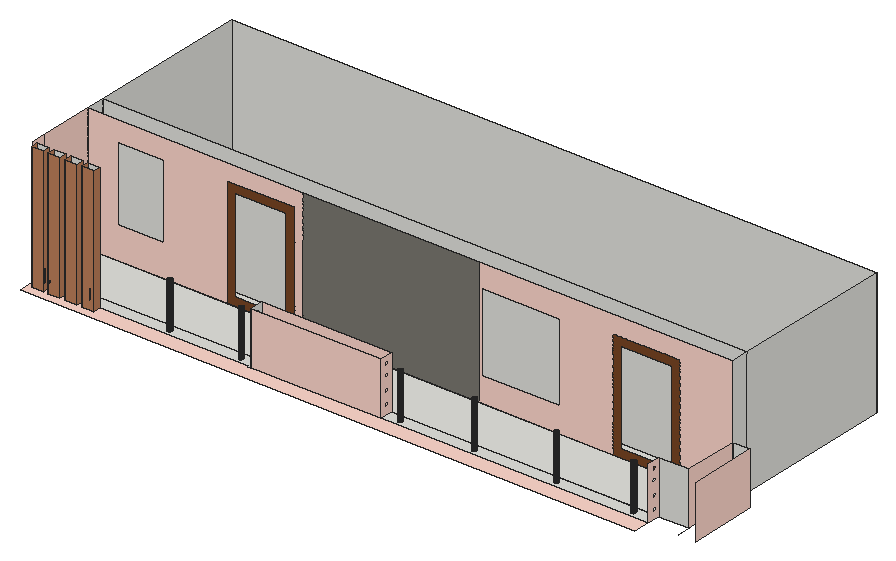
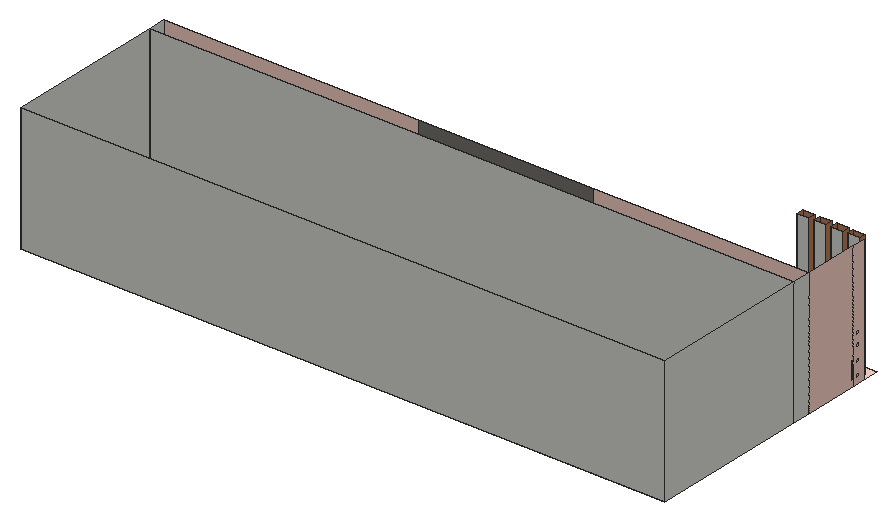
# SketchUp Ruby script. Lengths in inches.
U = 1.inch
M = Sketchup.active_model
def pt(a) = Geom::Point3d.new(a.map { |v| v * U })
def face(e, loops, mat)
  f = e.add_face(loops[0].map { |a| pt(a) })
  loops[1..].each { |l| e.add_face(l.map { |a| pt(a) }).erase! }
  f.material = f.back_material = mat if mat
  f
end
# faces: each face lists its corners as indices into pts; further lists are holes
def faces(e, pts, list, mat = nil) = list.each { |f| face(e, (f[0].is_a?(Array) ? f : [f]).map { |l| l.map { |i| pts[i] } }, mat) }
# xy, xz, yz: faces in a plane at the given z, y or x. An outline is a flat list of corners, or four numbers for a rectangle; further outlines are holes
def ring(l) = l.size == 4 ? [[l[0], l[1]], [l[2], l[1]], [l[2], l[3]], [l[0], l[3]]] : l.each_slice(2).to_a
def flat(e, list, mat, &to3) = list.each { |f| face(e, (f[0].is_a?(Array) ? f : [f]).map { |l| ring(l).map { |u, v| to3.(u, v) } }, mat) }
def xy(e, z, list, mat = nil) = flat(e, list, mat) { |x, y| [x, y, z] }
def xz(e, y, list, mat = nil) = flat(e, list, mat) { |x, z| [x, y, z] }
def yz(e, x, list, mat = nil) = flat(e, list, mat) { |y, z| [x, y, z] }
def lines(e, pts, list) = list.each { |a, b| e.add_line(pt(pts[a]), pt(pts[b])) }
# prism: a flat outline (further loops are holes) pulled along v
def prism(e, loops, v, mat = nil)
  f = face(e, loops, mat); d = Geom::Vector3d.new(v.map { |x| x * U })
  f.pushpull(f.normal.samedirection?(d) ? d.length : -d.length)
end
def box(e, o, s, mat = nil) = prism(e, [[o, [o[0] + s[0], o[1], o[2]], [o[0] + s[0], o[1] + s[1], o[2]], [o[0], o[1] + s[1], o[2]]]], [0, 0, s[2]], mat)
def at(x, y, z, deg = 0) = Geom::Transformation.translation(pt([x, y, z])) * Geom::Transformation.rotation(ORIGIN, Z_AXIS, deg.degrees)
def axes(o, x, y, z) = Geom::Transformation.new([*x, 0, *y, 0, *z, 0, *pt(o).to_a, 1])
def part(name) = M.definitions.add(name)
# library, detail: a bought-in or finely detailed component or shape, given as its bounding box
def library(name, o, s) = part(name).tap { |d| box(d.entities, o, s) }
def detail(e, o, s) = box(e.add_group.entities, o, s)
def put(e, d, t, mat = nil) = e.add_instance(d, t).tap { |i| i.material = mat if mat }
def group(e, t, mat = nil) = e.add_group.tap { |g| g.transformation = t; g.material = mat if mat }.entities
root = M.entities
M.materials.add("[Color B01]").color = [255, 216, 204]
M.materials.add("[Rough Square Concrete Block]").color = [123, 120, 113]
M.materials.add("[Wood Veneer 01]1").color = [120, 70, 37]
M.materials.add("[Wood Veneer 02]").color = [190, 128, 91]
xy(root,1353.25,[[2027.68,288.33,2025.25,288.65,2022.99,289.59,2021.05,291.08,2019.5625,293.02,2018.625,295.28,2018.31,297.71,2018.625,300.13,2019.5625,302.39,2021.05,304.34,2022.99,305.83,2025.25,306.76,2027.68,307.08,2030.11,306.76,2032.37,305.83,2034.31,304.34,2035.8,302.39,2036.74,300.13,2037.06,297.71,2036.74,295.28,2035.8,293.02,2034.31,291.08,2032.37,289.59,2030.11,288.65]])
xy(root,1357.0625,[[[77.93,267.5625,1053.15,328.8],[116.87,288.33,114.44,288.65,112.18,289.59,110.24,291.08,108.75,293.02,107.8125,295.28,107.49,297.71,107.8125,300.13,108.75,302.39,110.24,304.34,112.18,305.83,114.44,306.76,116.87,307.08,119.3,306.76,121.56,305.83,123.5,304.34,124.99,302.39,125.92,300.13,126.24,297.71,125.92,295.28,124.99,293.02,123.5,291.08,121.56,289.59,119.3,288.65],[984.12,288.33,981.69,288.65,979.43,289.59,977.49,291.08,976,293.02,975.0625,295.28,974.74,297.71,975.0625,300.13,976,302.39,977.49,304.34,979.43,305.83,981.69,306.76,984.12,307.08,986.55,306.76,988.81,305.83,990.75,304.34,992.24,302.39,993.17,300.13,993.49,297.71,993.17,295.28,992.24,293.02,990.75,291.08,988.81,289.59,986.55,288.65],[319.87,288.33,317.44,288.65,315.18,289.59,313.24,291.08,311.75,293.02,310.8125,295.28,310.49,297.71,310.8125,300.13,311.75,302.39,313.24,304.34,315.18,305.83,317.44,306.76,319.87,307.08,322.3,306.76,324.56,305.83,326.5,304.34,327.99,302.39,328.92,300.13,329.24,297.71,328.92,295.28,327.99,293.02,326.5,291.08,324.56,289.59,322.3,288.65],[664.37,288.33,661.94,288.65,659.68,289.59,657.74,291.08,656.25,293.02,655.3125,295.28,654.99,297.71,655.3125,300.13,656.25,302.39,657.74,304.34,659.68,305.83,661.94,306.76,664.37,307.08,666.8,306.76,669.06,305.83,671,304.34,672.49,302.39,673.42,300.13,673.74,297.71,673.42,295.28,672.49,293.02,671,291.08,669.06,289.59,666.8,288.65]],[1053.15,267.5625,1631.4,328.8],[[1631.4,267.5625,2829.41,328.8],[2740.43,288.33,2738,288.65,2735.74,289.59,2733.8,291.08,2732.3125,293.02,2731.375,295.28,2731.06,297.71,2731.375,300.13,2732.3125,302.39,2733.8,304.34,2735.74,305.83,2738,306.76,2740.43,307.08,2742.86,306.76,2745.12,305.83,2747.06,304.34,2748.55,302.39,2749.49,300.13,2749.81,297.71,2749.49,295.28,2748.55,293.02,2747.06,291.08,2745.12,289.59,2742.86,288.65],[1696.31,288.33,1693.88,288.65,1691.62,289.59,1689.68,291.08,1688.1875,293.02,1687.25,295.28,1686.93,297.71,1687.25,300.13,1688.1875,302.39,1689.68,304.34,1691.62,305.83,1693.88,306.76,1696.31,307.08,1698.73,306.76,1700.99,305.83,1702.94,304.34,1704.43,302.39,1705.36,300.13,1705.68,297.71,1705.36,295.28,1704.43,293.02,1702.94,291.08,1700.99,289.59,1698.73,288.65],[2395.24,288.33,2392.82,288.65,2390.56,289.59,2388.61,291.08,2387.125,293.02,2386.1875,295.28,2385.87,297.71,2386.1875,300.13,2387.125,302.39,2388.61,304.34,2390.56,305.83,2392.82,306.76,2395.24,307.08,2397.67,306.76,2399.93,305.83,2401.87,304.34,2403.36,302.39,2404.3,300.13,2404.62,297.71,2404.3,295.28,2403.36,293.02,2401.87,291.08,2399.93,289.59,2397.67,288.65],[2027.68,288.33,2025.25,288.65,2022.99,289.59,2021.05,291.08,2019.5625,293.02,2018.625,295.28,2018.31,297.71,2018.625,300.13,2019.5625,302.39,2021.05,304.34,2022.99,305.83,2025.25,306.76,2027.68,307.08,2030.11,306.76,2032.37,305.83,2034.31,304.34,2035.8,302.39,2036.74,300.13,2037.06,297.71,2036.74,295.28,2035.8,293.02,2034.31,291.08,2032.37,289.59,2030.11,288.65]],[116.87,288.33,114.44,288.65,112.18,289.59,110.24,291.08,108.75,293.02,107.8125,295.28,107.49,297.71,107.8125,300.13,108.75,302.39,110.24,304.34,112.18,305.83,114.44,306.76,116.87,307.08,119.3,306.76,121.56,305.83,123.5,304.34,124.99,302.39,125.92,300.13,126.24,297.71,125.92,295.28,124.99,293.02,123.5,291.08,121.56,289.59,119.3,288.65],[319.87,288.33,317.44,288.65,315.18,289.59,313.24,291.08,311.75,293.02,310.8125,295.28,310.49,297.71,310.8125,300.13,311.75,302.39,313.24,304.34,315.18,305.83,317.44,306.76,319.87,307.08,322.3,306.76,324.56,305.83,326.5,304.34,327.99,302.39,328.92,300.13,329.24,297.71,328.92,295.28,327.99,293.02,326.5,291.08,324.56,289.59,322.3,288.65],
  [664.37,288.33,661.94,288.65,659.68,289.59,657.74,291.08,656.25,293.02,655.3125,295.28,654.99,297.71,655.3125,300.13,656.25,302.39,657.74,304.34,659.68,305.83,661.94,306.76,664.37,307.08,666.8,306.76,669.06,305.83,671,304.34,672.49,302.39,673.42,300.13,673.74,297.71,673.42,295.28,672.49,293.02,671,291.08,669.06,289.59,666.8,288.65],[984.12,288.33,981.69,288.65,979.43,289.59,977.49,291.08,976,293.02,975.0625,295.28,974.74,297.71,975.0625,300.13,976,302.39,977.49,304.34,979.43,305.83,981.69,306.76,984.12,307.08,986.55,306.76,988.81,305.83,990.75,304.34,992.24,302.39,993.17,300.13,993.49,297.71,993.17,295.28,992.24,293.02,990.75,291.08,988.81,289.59,986.55,288.65],[1696.31,288.33,1693.88,288.65,1691.62,289.59,1689.68,291.08,1688.1875,293.02,1687.25,295.28,1686.93,297.71,1687.25,300.13,1688.1875,302.39,1689.68,304.34,1691.62,305.83,1693.88,306.76,1696.31,307.08,1698.73,306.76,1700.99,305.83,1702.94,304.34,1704.43,302.39,1705.36,300.13,1705.68,297.71,1705.36,295.28,1704.43,293.02,1702.94,291.08,1700.99,289.59,1698.73,288.65],[2027.68,288.33,2025.25,288.65,2022.99,289.59,2021.05,291.08,2019.5625,293.02,2018.625,295.28,2018.31,297.71,2018.625,300.13,2019.5625,302.39,2021.05,304.34,2022.99,305.83,2025.25,306.76,2027.68,307.08,2030.11,306.76,2032.37,305.83,2034.31,304.34,2035.8,302.39,2036.74,300.13,2037.06,297.71,2036.74,295.28,2035.8,293.02,2034.31,291.08,2032.37,289.59,2030.11,288.65],[2395.24,288.33,2392.82,288.65,2390.56,289.59,2388.61,291.08,2387.125,293.02,2386.1875,295.28,2385.87,297.71,2386.1875,300.13,2387.125,302.39,2388.61,304.34,2390.56,305.83,2392.82,306.76,2395.24,307.08,2397.67,306.76,2399.93,305.83,2401.87,304.34,2403.36,302.39,2404.3,300.13,2404.62,297.71,2404.3,295.28,2403.36,293.02,2401.87,291.08,2399.93,289.59,2397.67,288.65],
  [2740.43,288.33,2738,288.65,2735.74,289.59,2733.8,291.08,2732.3125,293.02,2731.375,295.28,2731.06,297.71,2731.375,300.13,2732.3125,302.39,2733.8,304.34,2735.74,305.83,2738,306.76,2740.43,307.08,2742.86,306.76,2745.12,305.83,2747.06,304.34,2748.55,302.39,2749.49,300.13,2749.81,297.71,2749.49,295.28,2748.55,293.02,2747.06,291.08,2745.12,289.59,2742.86,288.65],[77.93,328.8,2962.22,571.9],[77.93,571.9,2962.22,653.97],[77.93,653.97,2962.22,1377.24]])
xy(root,1357.0625,[[77.93,195.0625,2829.41,195.0625,2829.41,267.5625,374.06,267.5625,374.06,236.1875,321,236.1875,321,267.5625,299,267.5625,299,236.1875,245.93,236.1875,245.93,267.5625,223.06,267.5625,223.06,236.1875,170,236.1875,170,267.5625,148.18,267.5625,148.18,236.1875,95.12,236.1875,95.12,267.5625,77.93,267.5625]],"[Color B01]")
xz(root,236.1875,[[95.12,1357.0625,148.18,1920.4375],[170,1357.0625,223.06,1920.4375],[245.93,1357.0625,299,1920.4375],[321,1357.0625,374.06,1920.4375]],"[Wood Veneer 02]")
xz(root,267.5625,[[95.12,1357.0625,148.18,1920.4375],[170,1357.0625,223.06,1920.4375],[245.93,1357.0625,299,1920.4375],[321,1357.0625,374.06,1920.4375]])
xz(root,267.5625,[[1053.15,1357.0625,1631.4,1594.125]],"[Color B01]")
xz(root,328.8,[[2829.41,1357.0625,2962.22,1594.125]])
xz(root,328.8,[[1053.15,1357.0625,1631.4,1594.125]],"[Color B01]")
xz(root,571.9,[[2962.22,1357.0625,3040.15,1594.125]])
xz(root,571.9,[[[77.93,1357.0625,699.45,1357.0625,699.45,1848.03,1002.89,1848.03,1002.89,1357.0625,1038.88,1357.0625,1038.88,1920.4375,77.93,1920.4375],[211.19,1500.46,417.32,1833.98]],[[1828.6875,1357.0625,2426.53,1357.0625,2426.53,1841.76,2726.09,1841.76,2726.09,1357.0625,2962.22,1357.0625,2962.22,1920.4375,1828.6875,1920.4375],[1839.4375,1468.18,2191.5,1820.24]]],"[Color B01]")
xz(root,571.9,[[1038.88,1357.0625,1828.6875,1920.4375]],"[Rough Square Concrete Block]")
xz(root,571.9,[[[699.45,1357.0625,1002.89,1848.03],[735.89,1393.5,966.45,1811.59]],[[2426.53,1357.0625,2726.09,1841.76],[2462.81,1393.34,2689.8125,1805.49]]],"[Wood Veneer 01]1")
xz(root,653.97,[[77.93,1357.0625,2962.22,1920.4375]])
xz(root,1377.24,[[77.93,1357.0625,2962.22,1920.4375]])
yz(root,77.93,[[571.9,1357.0625,653.97,1920.4375],[653.97,1357.0625,1377.24,1920.4375]])
yz(root,77.93,[[[267.5625,1357.0625,328.8,1920.4375],[299.67,1381.78,297.25,1382.1,295.01,1383.03,293.08,1384.51,291.6,1386.4375,290.67,1388.68,290.35,1391.09,290.67,1393.5,291.6,1395.75,293.08,1397.68,295.01,1399.16,297.25,1400.09,299.67,1400.41,302.08,1400.09,304.32,1399.16,306.25,1397.68,307.73,1395.75,308.66,1393.5,308.98,1391.09,308.66,1388.68,307.73,1386.4375,306.25,1384.51,304.32,1383.03,302.08,1382.1],[299.67,1440.84,297.25,1441.16,295.01,1442.09,293.08,1443.57,291.6,1445.5,290.67,1447.74,290.35,1450.16,290.67,1452.57,291.6,1454.8125,293.08,1456.74,295.01,1458.22,297.25,1459.15,299.67,1459.47,302.08,1459.15,304.32,1458.22,306.25,1456.74,307.73,1454.8125,308.66,1452.57,308.98,1450.16,308.66,1447.74,307.73,1445.5,306.25,1443.57,304.32,1442.09,302.08,1441.16],[299.67,1504.28,297.25,1504.6,295.01,1505.53,293.08,1507.01,291.6,1508.9375,290.67,1511.18,290.35,1513.59,290.67,1516,291.6,1518.25,293.08,1520.18,295.01,1521.66,297.25,1522.59,299.67,1522.91,302.08,1522.59,304.32,1521.66,306.25,1520.18,307.73,1518.25,308.66,1516,308.98,1513.59,308.66,1511.18,307.73,1508.9375,306.25,1507.01,304.32,1505.53,302.08,1504.6],[299.67,1553.91,297.25,1554.22,295.01,1555.15,293.08,1556.63,291.6,1558.5625,290.67,1560.81,290.35,1563.22,290.67,1565.63,291.6,1567.875,293.08,1569.8,295.01,1571.28,297.25,1572.21,299.67,1572.53,302.08,1572.21,304.32,1571.28,306.25,1569.8,307.73,1567.875,308.66,1565.63,308.98,1563.22,308.66,1560.81,307.73,1558.5625,306.25,1556.63,304.32,1555.15,302.08,1554.22]],[328.8,1357.0625,571.9,1920.4375]],"[Color B01]")
yz(root,95.12,[[236.1875,1357.0625,267.5625,1920.4375]],"[Wood Veneer 02]")
yz(root,148.18,[[236.1875,1357.0625,267.5625,1920.4375]],"[Wood Veneer 02]")
yz(root,170,[[236.1875,1357.0625,267.5625,1920.4375]],"[Wood Veneer 02]")
yz(root,223.06,[[236.1875,1357.0625,267.5625,1920.4375]],"[Wood Veneer 02]")
yz(root,245.93,[[236.1875,1357.0625,267.5625,1920.4375]],"[Wood Veneer 02]")
yz(root,299,[[236.1875,1357.0625,267.5625,1920.4375]],"[Wood Veneer 02]")
yz(root,321,[[236.1875,1357.0625,267.5625,1920.4375]],"[Wood Veneer 02]")
yz(root,374.06,[[236.1875,1357.0625,267.5625,1920.4375]],"[Wood Veneer 02]")
yz(root,1053.15,[[[267.5625,1357.0625,328.8,1594.125],[299.67,1381.78,302.08,1382.1,304.32,1383.03,306.25,1384.51,307.73,1386.4375,308.66,1388.68,308.98,1391.09,308.66,1393.5,307.73,1395.75,306.25,1397.68,304.32,1399.16,302.08,1400.09,299.67,1400.41,297.25,1400.09,295.01,1399.16,293.08,1397.68,291.6,1395.75,290.67,1393.5,290.35,1391.09,290.67,1388.68,291.6,1386.4375,293.08,1384.51,295.01,1383.03,297.25,1382.1],[299.67,1504.28,302.08,1504.6,304.32,1505.53,306.25,1507.01,307.73,1508.9375,308.66,1511.18,308.98,1513.59,308.66,1516,307.73,1518.25,306.25,1520.18,304.32,1521.66,302.08,1522.59,299.67,1522.91,297.25,1522.59,295.01,1521.66,293.08,1520.18,291.6,1518.25,290.67,1516,290.35,1513.59,290.67,1511.18,291.6,1508.9375,293.08,1507.01,295.01,1505.53,297.25,1504.6],[299.67,1440.84,302.08,1441.16,304.32,1442.09,306.25,1443.57,307.73,1445.5,308.66,1447.74,308.98,1450.16,308.66,1452.57,307.73,1454.8125,306.25,1456.74,304.32,1458.22,302.08,1459.15,299.67,1459.47,297.25,1459.15,295.01,1458.22,293.08,1456.74,291.6,1454.8125,290.67,1452.57,290.35,1450.16,290.67,1447.74,291.6,1445.5,293.08,1443.57,295.01,1442.09,297.25,1441.16],[299.67,1553.91,302.08,1554.22,304.32,1555.15,306.25,1556.63,307.73,1558.5625,308.66,1560.81,308.98,1563.22,308.66,1565.63,307.73,1567.875,306.25,1569.8,304.32,1571.28,302.08,1572.21,299.67,1572.53,297.25,1572.21,295.01,1571.28,293.08,1569.8,291.6,1567.875,290.67,1565.63,290.35,1563.22,290.67,1560.81,291.6,1558.5625,293.08,1556.63,295.01,1555.15,297.25,1554.22]]])
yz(root,1631.4,[[[267.5625,1357.0625,328.8,1594.125],[299.67,1553.91,297.25,1554.22,295.01,1555.15,293.08,1556.63,291.6,1558.5625,290.67,1560.81,290.35,1563.22,290.67,1565.63,291.6,1567.875,293.08,1569.8,295.01,1571.28,297.25,1572.21,299.67,1572.53,302.08,1572.21,304.32,1571.28,306.25,1569.8,307.73,1567.875,308.66,1565.63,308.98,1563.22,308.66,1560.81,307.73,1558.5625,306.25,1556.63,304.32,1555.15,302.08,1554.22],[299.67,1507.03,297.25,1507.35,295.01,1508.28,293.08,1509.76,291.6,1511.6875,290.67,1513.93,290.35,1516.34,290.67,1518.75,291.6,1521,293.08,1522.93,295.01,1524.41,297.25,1525.34,299.67,1525.66,302.08,1525.34,304.32,1524.41,306.25,1522.93,307.73,1521,308.66,1518.75,308.98,1516.34,308.66,1513.93,307.73,1511.6875,306.25,1509.76,304.32,1508.28,302.08,1507.35],[299.67,1445.16,297.25,1445.47,295.01,1446.4,293.08,1447.88,291.6,1449.8125,290.67,1452.06,290.35,1454.47,290.67,1456.88,291.6,1459.125,293.08,1461.05,295.01,1462.53,297.25,1463.46,299.67,1463.78,302.08,1463.46,304.32,1462.53,306.25,1461.05,307.73,1459.125,308.66,1456.88,308.98,1454.47,308.66,1452.06,307.73,1449.8125,306.25,1447.88,304.32,1446.4,302.08,1445.47],[299.67,1388.28,297.25,1388.6,295.01,1389.53,293.08,1391.01,291.6,1392.9375,290.67,1395.18,290.35,1397.59,290.67,1400,291.6,1402.25,293.08,1404.18,295.01,1405.66,297.25,1406.59,299.67,1406.91,302.08,1406.59,304.32,1405.66,306.25,1404.18,307.73,1402.25,308.66,1400,308.98,1397.59,308.66,1395.18,307.73,1392.9375,306.25,1391.01,304.32,1389.53,302.08,1388.6]]],"[Color B01]")
yz(root,2829.41,[[[267.5625,1357.0625,328.8,1594.125],[299.67,1553.91,302.08,1554.22,304.32,1555.15,306.25,1556.63,307.73,1558.5625,308.66,1560.81,308.98,1563.22,308.66,1565.63,307.73,1567.875,306.25,1569.8,304.32,1571.28,302.08,1572.21,299.67,1572.53,297.25,1572.21,295.01,1571.28,293.08,1569.8,291.6,1567.875,290.67,1565.63,290.35,1563.22,290.67,1560.81,291.6,1558.5625,293.08,1556.63,295.01,1555.15,297.25,1554.22],[299.67,1388.28,302.08,1388.6,304.32,1389.53,306.25,1391.01,307.73,1392.9375,308.66,1395.18,308.98,1397.59,308.66,1400,307.73,1402.25,306.25,1404.18,304.32,1405.66,302.08,1406.59,299.67,1406.91,297.25,1406.59,295.01,1405.66,293.08,1404.18,291.6,1402.25,290.67,1400,290.35,1397.59,290.67,1395.18,291.6,1392.9375,293.08,1391.01,295.01,1389.53,297.25,1388.6],[299.67,1507.03,302.08,1507.35,304.32,1508.28,306.25,1509.76,307.73,1511.6875,308.66,1513.93,308.98,1516.34,308.66,1518.75,307.73,1521,306.25,1522.93,304.32,1524.41,302.08,1525.34,299.67,1525.66,297.25,1525.34,295.01,1524.41,293.08,1522.93,291.6,1521,290.67,1518.75,290.35,1516.34,290.67,1513.93,291.6,1511.6875,293.08,1509.76,295.01,1508.28,297.25,1507.35],[299.67,1445.16,302.08,1445.47,304.32,1446.4,306.25,1447.88,307.73,1449.8125,308.66,1452.06,308.98,1454.47,308.66,1456.88,307.73,1459.125,306.25,1461.05,304.32,1462.53,302.08,1463.46,299.67,1463.78,297.25,1463.46,295.01,1462.53,293.08,1461.05,291.6,1459.125,290.67,1456.88,290.35,1454.47,290.67,1452.06,291.6,1449.8125,293.08,1447.88,295.01,1446.4,297.25,1445.47]]],"[Color B01]")
yz(root,2962.22,[[571.9,1357.0625,653.97,1920.4375],[653.97,1357.0625,1377.24,1920.4375]])
yz(root,2962.22,[[328.8,1357.0625,571.9,1594.125]],"[Color B01]")
yz(root,3040.15,[[267.5625,1357.0625,571.9,1594.125]],"[Color B01]")
p = [[2027.68,288.33,1357.0625],[2025.25,288.65,1357.0625],[2025.25,288.65,1353.25],[2027.68,288.33,1353.25],[2030.11,288.65,1357.0625],[2030.11,288.65,1353.25],
  [2022.99,289.59,1357.0625],[2022.99,289.59,1353.25],[2032.37,289.59,1357.0625],[2032.37,289.59,1353.25],[2021.05,291.08,1357.0625],[2021.05,291.08,1353.25],
  [2034.31,291.08,1357.0625],[2034.31,291.08,1353.25],[2019.5625,293.02,1357.0625],[2019.5625,293.02,1353.25],[2035.8,293.02,1357.0625],[2035.8,293.02,1353.25],
  [2018.625,295.28,1357.0625],[2018.625,295.28,1353.25],[2036.74,295.28,1357.0625],[2036.74,295.28,1353.25],[2018.31,297.71,1357.0625],[2018.31,297.71,1353.25],
  [2037.06,297.71,1357.0625],[2037.06,297.71,1353.25],[2018.625,300.13,1357.0625],[2018.625,300.13,1353.25],[2036.74,300.13,1357.0625],[2036.74,300.13,1353.25],
  [2019.5625,302.39,1357.0625],[2019.5625,302.39,1353.25],[2035.8,302.39,1357.0625],[2035.8,302.39,1353.25],[2021.05,304.34,1357.0625],[2021.05,304.34,1353.25],
  [2034.31,304.34,1357.0625],[2034.31,304.34,1353.25],[2022.99,305.83,1357.0625],[2022.99,305.83,1353.25],[2032.37,305.83,1357.0625],[2032.37,305.83,1353.25],
  [2025.25,306.76,1357.0625],[2025.25,306.76,1353.25],[2030.11,306.76,1357.0625],[2030.11,306.76,1353.25],[2027.68,307.08,1357.0625],[2027.68,307.08,1353.25],
  [114.44,288.65,1357.0625],[116.87,288.33,1357.0625],[116.87,288.33,1561],[114.44,288.65,1561],[119.3,288.65,1357.0625],[119.3,288.65,1561],
  [317.44,288.65,1357.0625],[319.87,288.33,1357.0625],[319.87,288.33,1564.4375],[317.44,288.65,1564.4375],[322.3,288.65,1357.0625],[322.3,288.65,1564.4375],
  [661.94,288.65,1357.0625],[664.37,288.33,1357.0625],[664.37,288.33,1561.375],[661.94,288.65,1561.375],[666.8,288.65,1357.0625],[666.8,288.65,1561.375],
  [981.69,288.65,1357.0625],[984.12,288.33,1357.0625],[984.12,288.33,1563.22],[981.69,288.65,1563.22],[986.55,288.65,1357.0625],[986.55,288.65,1563.22],
  [1693.88,288.65,1357.0625],[1696.31,288.33,1357.0625],[1696.31,288.33,1559.8125],[1693.88,288.65,1559.8125],[1698.73,288.65,1357.0625],[1698.73,288.65,1559.8125],
  [2027.68,288.33,1563.8125],[2025.25,288.65,1563.8125],[2030.11,288.65,1563.8125],[2392.82,288.65,1357.0625],[2395.24,288.33,1357.0625],[2395.24,288.33,1560.375],
  [2392.82,288.65,1560.375],[2397.67,288.65,1357.0625],[2397.67,288.65,1560.375],[2738,288.65,1357.0625],[2740.43,288.33,1357.0625],[2740.43,288.33,1562.5625],
  [2738,288.65,1562.5625],[2742.86,288.65,1357.0625],[2742.86,288.65,1562.5625],[112.18,289.59,1357.0625],[112.18,289.59,1561],[121.56,289.59,1357.0625],
  [121.56,289.59,1561],[315.18,289.59,1357.0625],[315.18,289.59,1564.4375],[324.56,289.59,1357.0625],[324.56,289.59,1564.4375],[659.68,289.59,1357.0625],
  [659.68,289.59,1561.375],[669.06,289.59,1357.0625],[669.06,289.59,1561.375],[979.43,289.59,1357.0625],[979.43,289.59,1563.22],[988.81,289.59,1357.0625],
  [988.81,289.59,1563.22],[1691.62,289.59,1357.0625],[1691.62,289.59,1559.8125],[1700.99,289.59,1357.0625],[1700.99,289.59,1559.8125],[2022.99,289.59,1563.8125],
  [2032.37,289.59,1563.8125],[2390.56,289.59,1357.0625],[2390.56,289.59,1560.375],[2399.93,289.59,1357.0625],[2399.93,289.59,1560.375],[2735.74,289.59,1357.0625],
  [2735.74,289.59,1562.5625],[2745.12,289.59,1357.0625],[2745.12,289.59,1562.5625],[110.24,291.08,1357.0625],[110.24,291.08,1561],[123.5,291.08,1357.0625],
  [123.5,291.08,1561],[313.24,291.08,1357.0625],[313.24,291.08,1564.4375],[326.5,291.08,1357.0625],[326.5,291.08,1564.4375],[657.74,291.08,1357.0625],
  [657.74,291.08,1561.375],[671,291.08,1357.0625],[671,291.08,1561.375],[977.49,291.08,1357.0625],[978.43,290.35,1563.22],[977.49,291.08,1563.22],
  [990.75,291.08,1357.0625],[990.75,291.08,1563.22],[989.8,290.35,1563.22],[1689.68,291.08,1357.0625],[1689.68,291.08,1559.8125],[1702.94,291.08,1357.0625],
  [1702.94,291.08,1559.8125],[2021.05,291.08,1563.8125],[2034.31,291.08,1563.8125],[2388.61,291.08,1357.0625],[2388.61,291.08,1560.375],[2401.87,291.08,1357.0625],
  [2401.87,291.08,1560.375],[2733.8,291.08,1357.0625],[2733.8,291.08,1562.5625],[2747.06,291.08,1357.0625],[2747.06,291.08,1562.5625],[108.75,293.02,1357.0625],
  [108.75,293.02,1561],[124.99,293.02,1357.0625],[124.99,293.02,1561],[311.75,293.02,1357.0625],[311.75,293.02,1564.4375],[327.99,293.02,1357.0625],
  [327.99,293.02,1564.4375],[656.25,293.02,1357.0625],[656.25,293.02,1561.375],[672.49,293.02,1357.0625],[672.49,293.02,1561.375],[976,293.02,1357.0625],
  [976,293.02,1563.22],[992.24,293.02,1357.0625],[992.24,293.02,1563.22],[1688.1875,293.02,1357.0625],[1688.1875,293.02,1559.8125],[1704.43,293.02,1357.0625],
  [1704.43,293.02,1559.8125],[2019.5625,293.02,1563.8125],[2035.8,293.02,1563.8125],[2387.125,293.02,1357.0625],[2387.125,293.02,1560.375],[2403.36,293.02,1357.0625],
  [2403.36,293.02,1560.375],[2732.3125,293.02,1357.0625],[2732.3125,293.02,1562.5625],[2748.55,293.02,1357.0625],[2748.55,293.02,1562.5625],[107.8125,295.28,1357.0625],
  [107.8125,295.28,1561],[125.92,295.28,1357.0625],[125.92,295.28,1561],[310.8125,295.28,1357.0625],[310.8125,295.28,1564.4375],[328.92,295.28,1357.0625],
  [328.92,295.28,1564.4375],[655.3125,295.28,1357.0625],[655.3125,295.28,1561.375],[673.42,295.28,1357.0625],[673.42,295.28,1561.375],[975.0625,295.28,1357.0625],
  [975.0625,295.28,1563.22],[993.17,295.28,1357.0625],[993.17,295.28,1563.22],[1687.25,295.28,1357.0625],[1687.25,295.28,1559.8125],[1705.36,295.28,1357.0625],
  [1705.36,295.28,1559.8125],[2018.625,295.28,1563.8125],[2036.74,295.28,1563.8125],[2386.1875,295.28,1357.0625],[2386.1875,295.28,1560.375],[2404.3,295.28,1357.0625],
  [2404.3,295.28,1560.375],[2731.375,295.28,1357.0625],[2731.375,295.28,1562.5625],[2749.49,295.28,1357.0625],[2749.49,295.28,1562.5625],[107.49,297.71,1357.0625],
  [107.49,297.71,1561],[126.24,297.71,1357.0625],[126.24,297.71,1561],[310.49,297.71,1357.0625],[310.49,297.71,1564.4375],[329.24,297.71,1357.0625],
  [329.24,297.71,1564.4375],[654.99,297.71,1357.0625],[654.99,297.71,1561.375],[673.74,297.71,1357.0625],[673.74,297.71,1561.375],[974.74,297.71,1357.0625],
  [974.74,297.71,1563.22],[993.49,297.71,1357.0625],[993.49,297.71,1563.22],[1686.93,297.71,1357.0625],[1686.93,297.71,1559.8125],[1705.68,297.71,1357.0625],
  [1705.68,297.71,1559.8125],[2018.31,297.71,1563.8125],[2037.06,297.71,1563.8125],[2385.87,297.71,1357.0625],[2385.87,297.71,1560.375],[2404.62,297.71,1357.0625],
  [2404.62,297.71,1560.375],[2731.06,297.71,1357.0625],[2731.06,297.71,1562.5625],[2749.81,297.71,1357.0625],[2749.81,297.71,1562.5625],[107.8125,300.13,1357.0625],
  [107.8125,300.13,1561],[125.92,300.13,1357.0625],[125.92,300.13,1561],[310.8125,300.13,1357.0625],[310.8125,300.13,1564.4375],[328.92,300.13,1357.0625],
  [328.92,300.13,1564.4375],[655.3125,300.13,1357.0625],[655.3125,300.13,1561.375],[673.42,300.13,1357.0625],[673.42,300.13,1561.375],[975.0625,300.13,1357.0625],
  [975.0625,300.13,1563.22],[993.17,300.13,1357.0625],[993.17,300.13,1563.22],[1687.25,300.13,1357.0625],[1687.25,300.13,1559.8125],[1705.36,300.13,1357.0625],
  [1705.36,300.13,1559.8125],[2018.625,300.13,1563.8125],[2036.74,300.13,1563.8125],[2386.1875,300.13,1357.0625],[2386.1875,300.13,1560.375],[2404.3,300.13,1357.0625],
  [2404.3,300.13,1560.375],[2731.375,300.13,1357.0625],[2731.375,300.13,1562.5625],[2749.49,300.13,1357.0625],[2749.49,300.13,1562.5625],[108.75,302.39,1357.0625],
  [108.75,302.39,1561],[124.99,302.39,1357.0625],[124.99,302.39,1561],[311.75,302.39,1357.0625],[311.75,302.39,1564.4375],[327.99,302.39,1357.0625],
  [327.99,302.39,1564.4375],[656.25,302.39,1357.0625],[656.25,302.39,1561.375],[672.49,302.39,1357.0625],[672.49,302.39,1561.375],[976,302.39,1357.0625],
  [976,302.39,1563.22],[992.24,302.39,1357.0625],[992.24,302.39,1563.22],[1688.1875,302.39,1357.0625],[1688.1875,302.39,1559.8125],[1704.43,302.39,1357.0625],
  [1704.43,302.39,1559.8125],[2019.5625,302.39,1563.8125],[2035.8,302.39,1563.8125],[2387.125,302.39,1357.0625],[2387.125,302.39,1560.375],[2403.36,302.39,1357.0625],
  [2403.36,302.39,1560.375],[2732.3125,302.39,1357.0625],[2732.3125,302.39,1562.5625],[2748.55,302.39,1357.0625],[2748.55,302.39,1562.5625],[110.24,304.34,1357.0625],
  [110.24,304.34,1561],[123.5,304.34,1357.0625],[123.5,304.34,1561],[313.24,304.34,1357.0625],[313.24,304.34,1564.4375],[326.5,304.34,1357.0625],
  [326.5,304.34,1564.4375],[657.74,304.34,1357.0625],[657.74,304.34,1561.375],[671,304.34,1357.0625],[671,304.34,1561.375],[977.49,304.34,1357.0625],
  [977.49,304.34,1563.22],[990.75,304.34,1357.0625],[990.75,304.34,1563.22],[1689.68,304.34,1357.0625],[1689.68,304.34,1559.8125],[1702.94,304.34,1357.0625],
  [1702.94,304.34,1559.8125],[2021.05,304.34,1563.8125],[2034.31,304.34,1563.8125],[2388.61,304.34,1357.0625],[2388.61,304.34,1560.375],[2401.87,304.34,1357.0625],
  [2401.87,304.34,1560.375],[2733.8,304.34,1357.0625],[2733.8,304.34,1562.5625],[2747.06,304.34,1357.0625],[2747.06,304.34,1562.5625],[112.18,305.83,1357.0625],
  [112.18,305.83,1561],[121.56,305.83,1357.0625],[121.56,305.83,1561],[315.18,305.83,1357.0625],[315.18,305.83,1564.4375],[324.56,305.83,1357.0625],
  [324.56,305.83,1564.4375],[659.68,305.83,1357.0625],[659.68,305.83,1561.375],[669.06,305.83,1357.0625],[669.06,305.83,1561.375],[979.43,305.83,1357.0625],
  [979.43,305.83,1563.22],[988.81,305.83,1357.0625],[988.81,305.83,1563.22],[1691.62,305.83,1357.0625],[1691.62,305.83,1559.8125],[1700.99,305.83,1357.0625],
  [1700.99,305.83,1559.8125],[2022.99,305.83,1563.8125],[2032.37,305.83,1563.8125],[2390.56,305.83,1357.0625],[2390.56,305.83,1560.375],[2399.93,305.83,1357.0625],
  [2399.93,305.83,1560.375],[2735.74,305.83,1357.0625],[2735.74,305.83,1562.5625],[2745.12,305.83,1357.0625],[2745.12,305.83,1562.5625],[114.44,306.76,1357.0625],
  [114.44,306.76,1561],[119.3,306.76,1357.0625],[119.3,306.76,1561],[317.44,306.76,1357.0625],[317.44,306.76,1564.4375],[322.3,306.76,1357.0625],
  [322.3,306.76,1564.4375],[661.94,306.76,1357.0625],[661.94,306.76,1561.375],[666.8,306.76,1357.0625],[666.8,306.76,1561.375],[981.69,306.76,1357.0625],
  [981.69,306.76,1563.22],[986.55,306.76,1357.0625],[986.55,306.76,1563.22],[1693.88,306.76,1357.0625],[1693.88,306.76,1559.8125],[1698.73,306.76,1357.0625],
  [1698.73,306.76,1559.8125],[2025.25,306.76,1563.8125],[2030.11,306.76,1563.8125],[2392.82,306.76,1357.0625],[2392.82,306.76,1560.375],[2397.67,306.76,1357.0625],
  [2397.67,306.76,1560.375],[2738,306.76,1357.0625],[2738,306.76,1562.5625],[2742.86,306.76,1357.0625],[2742.86,306.76,1562.5625],[116.87,307.08,1357.0625],
  [116.87,307.08,1561],[319.87,307.08,1357.0625],[319.87,307.08,1564.4375],[664.37,307.08,1357.0625],[664.37,307.08,1561.375],[984.12,307.08,1357.0625],
  [984.12,307.08,1563.22],[1696.31,307.08,1357.0625],[1696.31,307.08,1559.8125],[2027.68,307.08,1563.8125],[2395.24,307.08,1357.0625],[2395.24,307.08,1560.375],
  [2740.43,307.08,1357.0625],[2740.43,307.08,1562.5625],[2962.22,328.8,1357.0625],[2962.22,267.5625,1357.0625]]
faces(root,p,[[0,1,2,3],[4,0,3,5],[1,6,7,2],[8,4,5,9],[6,10,11,7],[12,8,9,13],[10,14,15,11],[16,12,13,17],
  [14,18,19,15],[20,16,17,21],[18,22,23,19],[24,20,21,25],[22,26,27,23],[28,24,25,29],[26,30,31,27],[32,28,29,33],
  [30,34,35,31],[36,32,33,37],[34,38,39,35],[40,36,37,41],[38,42,43,39],[44,40,41,45],[42,46,47,43],[46,44,45,47]])
faces(root,p,[[48,49,50,51],[49,52,53,50],[54,55,56,57],[55,58,59,56],[60,61,62,63],[61,64,65,62],[66,67,68,69],[67,70,71,68],
  [72,73,74,75],[73,76,77,74],[1,0,78,79],[0,4,80,78],[81,82,83,84],[82,85,86,83],[87,88,89,90],[88,91,92,89],
  [93,48,51,94],[52,95,96,53],[97,54,57,98],[58,99,100,59],[101,60,63,102],[64,103,104,65],[105,66,69,106],[70,107,108,71],
  [109,72,75,110],[76,111,112,77],[6,1,79,113],[4,8,114,80],[115,81,84,116],[85,117,118,86],[119,87,90,120],[91,121,122,92],
  [123,93,94,124],[95,125,126,96],[127,97,98,128],[99,129,130,100],[131,101,102,132],[103,133,134,104],[135,105,106,136,137],[107,138,139,140,108],
  [141,109,110,142],[111,143,144,112],[10,6,113,145],[8,12,146,114],[147,115,116,148],[117,149,150,118],[151,119,120,152],[121,153,154,122],
  [155,123,124,156],[125,157,158,126],[159,127,128,160],[129,161,162,130],[163,131,132,164],[133,165,166,134],[167,135,137,168],[138,169,170,139],
  [171,141,142,172],[143,173,174,144],[14,10,145,175],[12,16,176,146],[177,147,148,178],[149,179,180,150],[181,151,152,182],[153,183,184,154],
  [185,155,156,186],[157,187,188,158],[189,159,160,190],[161,191,192,162],[193,163,164,194],[165,195,196,166],[197,167,168,198],[169,199,200,170],
  [201,171,172,202],[173,203,204,174],[18,14,175,205],[16,20,206,176],[207,177,178,208],[179,209,210,180],[211,181,182,212],[183,213,214,184],
  [215,185,186,216],[187,217,218,188],[219,189,190,220],[191,221,222,192],[223,193,194,224],[195,225,226,196],[227,197,198,228],[199,229,230,200],
  [231,201,202,232],[203,233,234,204],[22,18,205,235],[20,24,236,206],[237,207,208,238],[209,239,240,210],[241,211,212,242],[213,243,244,214],
  [245,215,216,246],[217,247,248,218],[249,219,220,250],[221,251,252,222],[253,223,224,254],[225,255,256,226],[257,227,228,258],[229,259,260,230],
  [261,231,232,262],[233,263,264,234],[26,22,235,265],[24,28,266,236],[267,237,238,268],[239,269,270,240],[271,241,242,272],[243,273,274,244],
  [275,245,246,276],[247,277,278,248],[279,249,250,280],[251,281,282,252],[283,253,254,284],[255,285,286,256],[287,257,258,288],[259,289,290,260],
  [291,261,262,292],[263,293,294,264],[30,26,265,295],[28,32,296,266],[297,267,268,298],[269,299,300,270],[301,271,272,302],[273,303,304,274],
  [305,275,276,306],[277,307,308,278],[309,279,280,310],[281,311,312,282],[313,283,284,314],[285,315,316,286],[317,287,288,318],[289,319,320,290],
  [321,291,292,322],[293,323,324,294],[34,30,295,325],[32,36,326,296],[327,297,298,328],[299,329,330,300],[331,301,302,332],[303,333,334,304],
  [335,305,306,336],[307,337,338,308],[339,309,310,340],[311,341,342,312],[343,313,314,344],[315,345,346,316],[347,317,318,348],[319,349,350,320],
  [351,321,322,352],[323,353,354,324],[38,34,325,355],[36,40,356,326],[357,327,328,358],[329,359,360,330],[361,331,332,362],[333,363,364,334],
  [365,335,336,366],[337,367,368,338],[369,339,340,370],[341,371,372,342],[373,343,344,374],[345,375,376,346],[377,347,348,378],[349,379,380,350],
  [381,351,352,382],[353,383,384,354],[42,38,355,385],[40,44,386,356],[387,357,358,388],[359,389,390,360],[391,361,362,392],[363,393,394,364],
  [395,365,366,396],[367,395,396,368],[397,369,370,398],[371,397,398,372],[399,373,374,400],[375,399,400,376],[401,377,378,402],[379,401,402,380],
  [403,381,382,404],[383,403,404,384],[46,42,385,405],[44,46,405,386],[406,387,388,407],[389,406,407,390],[408,391,392,409],[393,408,409,394]],"[Wood Veneer 02]")
lines(root,p,[[410,411]])
